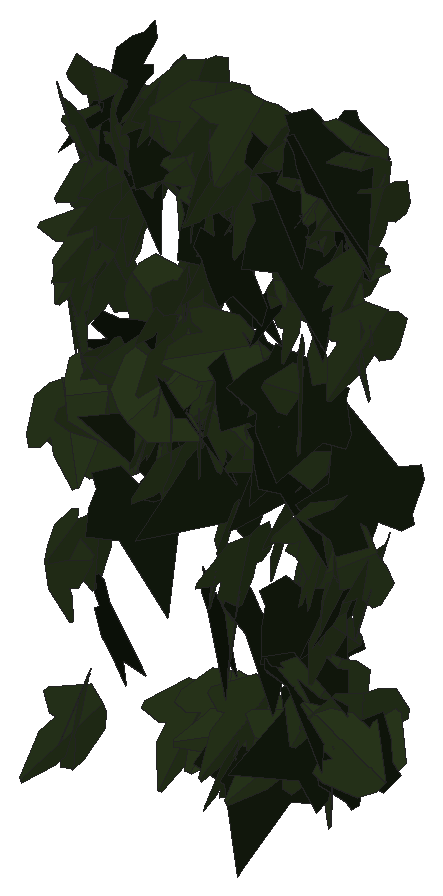
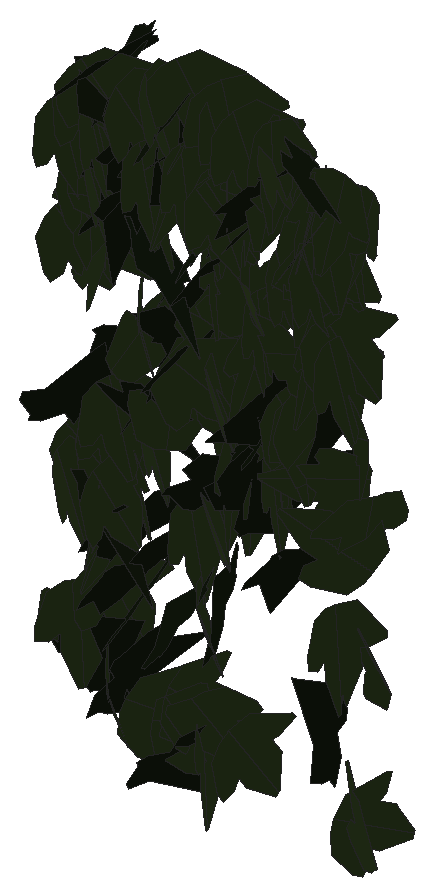
# SketchUp Ruby script. Lengths in inches.
U = 1.inch
M = Sketchup.active_model
def pt(a) = Geom::Point3d.new(a.map { |v| v * U })
def face(e, loops, mat)
  f = e.add_face(loops[0].map { |a| pt(a) })
  loops[1..].each { |l| e.add_face(l.map { |a| pt(a) }).erase! }
  f.material = f.back_material = mat if mat
  f
end
# faces: each face lists its corners as indices into pts; further lists are holes
def faces(e, pts, list, mat = nil) = list.each { |f| face(e, (f[0].is_a?(Array) ? f : [f]).map { |l| l.map { |i| pts[i] } }, mat) }
# xy, xz, yz: faces in a plane at the given z, y or x. An outline is a flat list of corners, or four numbers for a rectangle; further outlines are holes
def ring(l) = l.size == 4 ? [[l[0], l[1]], [l[2], l[1]], [l[2], l[3]], [l[0], l[3]]] : l.each_slice(2).to_a
def flat(e, list, mat, &to3) = list.each { |f| face(e, (f[0].is_a?(Array) ? f : [f]).map { |l| ring(l).map { |u, v| to3.(u, v) } }, mat) }
def xy(e, z, list, mat = nil) = flat(e, list, mat) { |x, y| [x, y, z] }
def xz(e, y, list, mat = nil) = flat(e, list, mat) { |x, z| [x, y, z] }
def yz(e, x, list, mat = nil) = flat(e, list, mat) { |y, z| [x, y, z] }
def lines(e, pts, list) = list.each { |a, b| e.add_line(pt(pts[a]), pt(pts[b])) }
# prism: a flat outline (further loops are holes) pulled along v
def prism(e, loops, v, mat = nil)
  f = face(e, loops, mat); d = Geom::Vector3d.new(v.map { |x| x * U })
  f.pushpull(f.normal.samedirection?(d) ? d.length : -d.length)
end
def box(e, o, s, mat = nil) = prism(e, [[o, [o[0] + s[0], o[1], o[2]], [o[0] + s[0], o[1] + s[1], o[2]], [o[0], o[1] + s[1], o[2]]]], [0, 0, s[2]], mat)
def at(x, y, z, deg = 0) = Geom::Transformation.translation(pt([x, y, z])) * Geom::Transformation.rotation(ORIGIN, Z_AXIS, deg.degrees)
def axes(o, x, y, z) = Geom::Transformation.new([*x, 0, *y, 0, *z, 0, *pt(o).to_a, 1])
def part(name) = M.definitions.add(name)
# library, detail: a bought-in or finely detailed component or shape, given as its bounding box
def library(name, o, s) = part(name).tap { |d| box(d.entities, o, s) }
def detail(e, o, s) = box(e.add_group.entities, o, s)
def put(e, d, t, mat = nil) = e.add_instance(d, t).tap { |i| i.material = mat if mat }
def group(e, t, mat = nil) = e.add_group.tap { |g| g.transformation = t; g.material = mat if mat }.entities
root = M.entities
M.materials.add("efeu1").color = [18, 25, 13]
M.materials.add("efeu2").color = [43, 57, 29]
c1 = part("ivyleaf_10")
p = [[0,0.5,-0.03],[-0.0625,2.02,-0.43],[-0.19,2.01,-0.46],[-0.54,1.05,-0.29],[-0.52,0.625,-0.18],[-0.83,0.76,-0.28],
  [-1.16,0.64,-0.33],[-1.15,0.33,-0.24],[-0.77,-0.39,0.02],[-0.3,-0.51,0.16],[0.04,-0.48,0.23],[-0.02,2.01,-0.4375],
  [-0.06,2.01,-0.43],[0.04,-0.49,0.23],[0.67,-0.49,0.14],[1.38,0.36,-0.2],[1.375,0.51,-0.24],[0.81,0.65,-0.19],
  [0.62,0.59,-0.15],[0.6,1.09,-0.28],[0.5,1.23,-0.31]]
faces(c1.entities,p,[[0,1,2,3,4,5,6,7,8,9,10],[11,12,0,13,14,15,16,17,18,19,20]],"efeu2")
c2 = part("ivyleaf_9")
p = [[1.54,2.16,1.25],[1.36,2.04,1.19],[-0.21,0.99,0.68],[-0.71,1.11,0.82],[-0.85,0.86,0.67],[-0.8,0.17,0.21],
  [-0.9,-0.01,0.1],[-0.67,-0.16,-0.02],[-0.08,-0.08,-0.05],[-0.03,-0.6,-0.4],[0.65,-0.88,-0.66],[0.83,-0.6,-0.49],
  [1.29,-0.42,-0.43],[1.8125,-0.07,-0.26],[1.21,0.44,0.15]]
faces(c2.entities,p,[[0,1,2,3,4,5,6,7,8,9,10,11,12,13,14]],"efeu1")
put(root,c1,axes([13.07,223.93,219.02],[0.34908,0.08349,-0.3481],[0.3274,0.12214,0.35762],[0.14475,-0.47761,0.0306]))
put(root,c2,axes([15.1,224.2,221.98],[-0.02137,-0.46964,-0.17023],[0.02814,0.16899,-0.46974],[0.49875,-0.02966,0.0192]))
put(root,c1,axes([11.76,224.47,214.32],[-0.03853,-0.20251,0.45553],[0.01998,-0.45714,-0.20154],[0.49811,0.00267,0.04332]))
put(root,c1,axes([14.96,224.19,218.31],[0.18515,-0.46397,0.0213],[0.00524,-0.02084,-0.49954],[0.46443,0.1852,-0.00286]))
put(root,c2,axes([14.79,224.2,218.98],[0.26219,-0.42405,-0.03791],[-0.02071,0.03177,-0.49856],[0.42524,0.26301,-0.00091]))
put(root,c2,axes([15.28,224.2,222.875],[0.32575,-0.3792,0.0098],[0.0052,-0.00845,-0.4999],[0.37929,0.32579,-0.00156]))
put(root,c1,axes([14.39,224.26,223.06],[-0.34984,-0.27143,0.23225],[-0.13064,-0.20535,-0.43677],[0.33248,-0.36628,0.07276]))
put(root,c1,axes([14.16,224.2,220.03],[0.19394,0.0032,-0.46085],[-0.4597,-0.03413,-0.19369],[-0.0327,0.49882,-0.0103]))
put(root,c1,axes([12.87,224.29,219.09],[0.37584,-0.28416,0.16732],[0.12516,-0.1118,-0.47099],[0.30509,0.39592,-0.01291]))
put(root,c2,axes([13.68,224.41,216.49],[0.13988,-0.0343,-0.47881],[0.44812,-0.16948,0.14305],[-0.17211,-0.46915,-0.01667]))
put(root,c1,axes([15.14,223.95,221.07],[0.15402,-0.15681,-0.4491],[-0.29345,0.3402,-0.21943],[0.37439,0.33117,0.01276]))
put(root,c1,axes([11.48,224.37,216.3],[0.1403,-0.18208,-0.44403],[0.33778,-0.29116,0.22612],[-0.34091,-0.36342,0.04131]))
put(root,c1,axes([15.47,224.25,218.32],[-0.16,-0.47044,0.05556],[-0.01054,-0.05509,-0.49684],[0.47359,-0.16016,0.00771]))
put(root,c1,axes([15.27,224.18,217.83],[0.33799,-0.34206,-0.13696],[-0.09006,0.10353,-0.4808],[0.35729,0.34968,0.00837]))
put(root,c2,axes([15,224.45,219.68],[-0.32889,-0.37655,0.00676],[-0.00644,-0.00335,-0.49995],[0.37655,-0.32894,-0.00264]))
put(root,c2,axes([13.98,224.1,221.375],[0.33709,-0.29994,-0.21542],[-0.1401,0.166,-0.45035],[0.34167,0.36398,0.02788]))
put(root,c1,axes([15.41,224.36,216.21],[-0.26685,-0.35438,0.23067],[-0.09339,-0.21663,-0.44085],[0.4124,-0.27836,0.04942]))
put(root,c1,axes([13.91,224.38,217.65],[0.29096,-0.37198,0.16423],[0.10235,-0.12843,-0.47226],[0.39353,0.30844,0.00141]))
put(root,c1,axes([15.98,224.3125,215.26],[0.27486,0.21407,0.35865],[-0.28049,-0.22353,0.34837],[0.30949,-0.3927,-0.00279]))
put(root,c1,axes([13.74,224.32,223.02],[-0.29322,-0.39187,0.10229],[-0.00417,-0.12336,-0.48453],[0.40498,-0.28499,0.06908]))
put(root,c2,axes([14.6,224.5,222.41],[0.12659,-0.43266,0.21628],[0.09311,-0.19759,-0.44977],[0.47466,0.15415,0.03054]))
put(root,c1,axes([13.28,224.23,220.375],[0.04579,-0.49298,-0.0698],[0.00656,0.07069,-0.49493],[0.49786,0.04441,0.01295]))
put(root,c1,axes([13.81,224.09,222.38],[0.15065,-0.38885,-0.27586],[-0.05128,0.27441,-0.41481],[0.474,0.15328,0.0428]))
put(root,c1,axes([13.46,224.21,220.4],[-0.11312,-0.46714,0.13779],[0.08053,0.12157,0.47826],[-0.48033,0.13039,0.04774]))
put(root,c1,axes([12.73,224.4375,219.34],[-0.07491,-0.45012,0.20439],[-0.02215,-0.20346,-0.45619],[0.49386,-0.07741,0.01054]))
put(root,c1,axes([13.81,224.3,222.8],[-0.00181,-0.49999,0.00153],[-0.00042,-0.00153,-0.5],[0.5,-0.00181,-0.00041]))
put(root,c1,axes([12.4375,224.29,221.76],[-0.35085,-0.13023,0.33158],[-0.31144,-0.11379,-0.37424],[0.17294,-0.46914,-0.00127]))
put(root,c2,axes([15.02,224.67,215.2],[0.09076,-0.28104,-0.40346],[0.12552,-0.38344,0.29533],[-0.4754,-0.15489,0.00095]))
put(root,c1,axes([13.36,224.21,218.33],[-0.10689,-0.47282,-0.12254],[0.03705,0.11723,-0.48465],[0.48703,-0.11268,0.00997]))
put(root,c1,axes([14.2,224.31,217.41],[-0.03852,-0.49843,-0.0092],[0.00113,0.00914,-0.49992],[0.49851,-0.03853,0.00042]))
put(root,c2,axes([14.83,224.5,216.21],[0.17024,-0.45509,0.11794],[0.0261,-0.11609,-0.48564],[0.4694,0.1715,-0.01577]))
put(root,c1,axes([13.68,224.44,218.96],[-0.09006,-0.04467,-0.48979],[0.41154,-0.27949,-0.05018],[-0.2693,-0.41218,0.08711]))
put(root,c2,axes([15.1,224.29,217.14],[0.07369,-0.42802,-0.24773],[-0.05304,0.24218,-0.4342],[0.49169,0.09027,-0.0097]))
put(root,c1,axes([14.09,224.62,215.23],[-0.05501,-0.30155,0.39502],[0.02432,-0.39859,-0.30089],[0.49637,-0.01389,0.05852]))
put(root,c1,axes([13.35,224.13,219.83],[-0.10307,-0.41364,-0.26129],[0.09995,0.2436,-0.42505],[0.47894,-0.13985,0.03247]))
put(root,c1,axes([15.71,224.53,221.49],[0.00181,-0.42673,0.26057],[0.01559,-0.2604,-0.42656],[0.49975,0.00967,0.01236]))
put(root,c2,axes([12.61,224.41,217.57],[0.03895,-0.47842,-0.13998],[0.01409,0.14141,-0.47938],[0.49828,0.0334,0.02449]))
put(root,c1,axes([14.71,224.41,222.83],[0.13065,-0.4775,0.07016],[0.01626,-0.06828,-0.49505],[0.48235,0.13164,-0.00231]))
put(root,c1,axes([11.8,224.21,222.2],[-0.42339,0.26533,0.01846],[-0.01493,0.01093,-0.49966],[-0.26556,-0.42365,-0.00133]))
put(root,c1,axes([12.44,224.26,221.375],[-0.11146,-0.47749,-0.09786],[0.00368,0.09956,-0.48997],[0.48741,-0.10994,-0.01868]))
put(root,c1,axes([11.99,224.5,220.65],[-0.22928,-0.35897,0.26187],[-0.08028,-0.25637,-0.4217],[0.43702,-0.23542,0.05992]))
put(root,c1,axes([12.41,224.66,219.05],[-0.08888,-0.19424,-0.45208],[-0.1362,-0.43173,0.21227],[-0.47281,0.16088,0.02383]))
put(root,c1,axes([15.88,224.53,220.77],[-0.13693,-0.40243,0.26326],[-0.0645,-0.25588,-0.4247],[0.47654,-0.15026,0.01816]))
put(root,c1,axes([12.91,224.5,222.75],[0.14554,-0.44777,0.16829],[0.04619,-0.16193,-0.47079],[0.47611,0.15259,-0.00577]))
put(root,c2,axes([15.33,224.46,223.08],[0.07842,-0.48579,-0.08863],[0.06513,0.09913,-0.48573],[0.4895,0.06464,0.07883]))
put(root,c1,axes([13.2,224.59,220.94],[0.21535,-0.17607,0.41548],[0.31437,-0.27172,-0.27809],[0.32372,0.38101,-0.00633]))
put(root,c2,axes([13.89,224.66,218.17],[-0.33893,-0.27039,0.24903],[-0.18704,-0.16476,-0.43344],[0.31645,-0.38697,0.01054]))
put(root,c1,axes([14.76,224.5625,219.84],[0.22591,-0.21738,0.3895],[0.32228,-0.2223,-0.31099],[0.30838,0.39157,0.03967]))
put(root,c1,axes([12.68,224.47,220.15],[-0.23664,-0.02364,-0.43982],[0.38833,-0.24681,-0.19566],[-0.20785,-0.4342,0.13517]))
put(root,c1,axes([14.64,224.67,214.92],[-0.13192,-0.20467,0.4367],[-0.07357,-0.43891,-0.22792],[0.47664,-0.12439,0.08568]))
put(root,c1,axes([13.02,224.3,222.42],[-0.43457,-0.24073,-0.05654],[0.04606,0.03353,-0.49674],[0.24295,-0.43695,-0.00697]))
put(root,c1,axes([15.86,224.38,217.85],[-0.27678,-0.01476,0.41614],[-0.40234,-0.11929,-0.27183],[0.10731,-0.48534,0.05416]))
put(root,c1,axes([13.06,224.22,219],[0.36545,-0.23482,-0.2476],[-0.11524,0.25655,-0.4134],[0.32119,0.35923,0.13339]))
put(root,c2,axes([13.0625,224.36,219.25],[0.39008,-0.30923,-0.04709],[-0.03417,0.0327,-0.49776],[0.31092,0.39155,0.00438]))
put(root,c1,axes([14.92,224.63,219.44],[-0.04595,0.29823,0.39868],[0.09084,-0.38864,0.30118],[0.48953,0.10011,-0.01847]))
put(root,c1,axes([11.55,224.48,214.08],[0.25014,-0.39273,-0.18218],[0.11358,-0.1435,0.4653],[-0.41777,-0.27417,0.01742]))
put(root,c1,axes([11.63,224.32,218.4],[0.19669,0.45876,0.0292],[0.01169,0.02676,-0.49915],[-0.45954,0.19704,-0.0002]))
put(root,c1,axes([13.25,224.66,214.9],[-0.13741,-0.37389,0.3022],[0.05814,-0.32492,-0.37556],[0.47722,-0.06807,0.13277]))
put(root,c1,axes([15.61,224.5625,222.62],[-0.15897,-0.43127,0.19681],[-0.03781,-0.19539,-0.45869],[0.47254,-0.16072,0.02951]))
put(root,c2,axes([15.51,224.23,222.64],[-0.20364,0.45648,0.01244],[-0.00547,0.01118,-0.49985],[-0.45662,-0.20371,0.00044]))
put(root,c1,axes([14.93,224.6,222.7],[-0.00767,-0.44717,0.22356],[-0.00255,-0.22354,-0.44724],[0.49993,-0.008,0.00115]))
put(root,c2,axes([12.39,224.21,219.51],[0.43256,0.05246,0.24524],[0.24385,0.02618,-0.43572],[-0.05856,0.49655,-0.00294]))
put(root,c1,axes([13.8,224.34,221.07],[0.04072,-0.47397,-0.15393],[-0.00353,0.15416,-0.47563],[0.49833,0.03982,0.00921]))
put(root,c1,axes([15.46,224.61,222.86],[-0.31299,-0.2872,0.26373],[-0.09033,-0.27558,-0.4073],[0.37932,-0.3026,0.12062]))
put(root,c1,axes([11.51,224.64,219.53],[-0.19426,0.14305,-0.43795],[0.23473,-0.37825,-0.22766],[-0.39644,-0.29405,0.0798]))
put(root,c2,axes([15.57,224.29,217.22],[-0.2818,0.40728,0.06866],[-0.04675,0.05114,-0.49518],[-0.41037,-0.2855,0.00926]))
put(root,c1,axes([15.45,224.18,216.98],[0.07593,-0.32824,-0.36945],[0.05396,0.37705,-0.32391],[0.49125,0.00932,0.09269]))
put(root,c1,axes([14.35,224.63,218.7],[-0.12286,-0.44473,-0.19267],[-0.06173,-0.18278,0.46128],[-0.48072,0.13713,-0.01]))
put(root,c1,axes([15.06,224.18,221.21],[0.01073,-0.13989,0.47991],[0.28537,0.39583,0.109],[-0.41043,0.27156,0.08834]))
put(root,c2,axes([14.93,224.63,221.59],[0.02893,-0.49827,-0.02976],[-0.00521,0.02951,-0.4991],[0.49914,0.02919,-0.00348]))
put(root,c1,axes([12.89,224.56,218.93],[0.43674,-0.21014,0.12288],[0.10673,-0.06154,-0.48458],[0.21879,0.4495,-0.00889]))
put(root,c2,axes([13.16,224.7,218.09],[-0.07589,-0.00901,0.49412],[-0.45574,-0.1921,-0.0735],[0.19116,-0.46154,0.02094]))
put(root,c1,axes([12.25,224.61,221.46],[0.01889,-0.47846,0.14393],[0.00629,-0.14379,-0.47884],[0.4996,0.0199,0.00058]))
put(root,c2,axes([14.95,224.58,216.64],[0.06157,-0.48432,-0.10788],[-0.0192,0.1063,-0.48819],[0.49582,0.06426,-0.00551]))
put(root,c2,axes([15.82,224.36,215.04],[0.07684,0.00598,0.49402],[-0.38099,0.31903,0.05539],[-0.31455,-0.38495,0.05358]))
put(root,c1,axes([15.19,224.54,218.73],[-0.18926,-0.45616,0.07808],[-0.02096,-0.07582,-0.49377],[0.46232,-0.19018,0.00957]))
put(root,c1,axes([12.49,224.48,219.38],[-0.11728,-0.48522,-0.02838],[-0.00332,0.03,-0.49909],[0.48604,-0.11688,-0.01026]))
put(root,c1,axes([14.03,224.7,219.54],[-0.18389,-0.2811,0.37036],[-0.19324,-0.31604,-0.33582],[0.4229,-0.26664,0.00759]))
put(root,c1,axes([12.23,224.49,221.96],[-0.46242,-0.1069,0.15729],[-0.13801,-0.09592,-0.47091],[0.13086,-0.47893,0.0592]))
put(root,c1,axes([15.48,224.53,222.25],[0.09386,-0.49109,-0.0048],[-0.00158,0.00459,-0.49998],[0.49111,0.09387,-0.00069]))
put(root,c1,axes([15.74,224.49,215.85],[-0.2909,-0.40652,0.01087],[-0.00523,-0.00963,-0.49988],[0.40663,-0.29094,0.00135]))
put(root,c1,axes([13.78,224.49,221.9],[0.02652,-0.49668,-0.05103],[0.01089,0.05167,-0.4972],[0.49918,0.02526,0.01356]))
put(root,c1,axes([12.44,224.31,222.34],[-0.17051,0.44273,0.15784],[-0.0954,0.13182,-0.47278],[-0.46025,-0.19134,0.03952]))
put(root,c1,axes([13.75,224.69,216.4],[0.30683,-0.28012,0.27818],[0.21003,-0.1825,-0.41543],[0.33428,0.37179,0.00567]))
put(root,c2,axes([14.14,224.46,219.67],[0.18861,-0.39686,-0.23859],[-0.0668,0.23161,-0.43806],[0.45822,0.19712,0.03435]))
put(root,c1,axes([15.6,224.48,220.88],[-0.14637,0.03623,0.47672],[-0.47421,-0.07442,-0.13995],[0.06081,-0.4931,0.05615]))
put(root,c1,axes([13.64,224.625,219.46],[0.26493,-0.41205,0.10014],[0.05252,-0.08528,-0.48987],[0.42078,0.27008,-0.0019]))
put(root,c1,axes([13.55,224.71,221.98],[-0.17957,-0.39272,0.25204],[-0.0255,-0.2614,-0.42547],[0.46595,-0.16565,0.07385]))
put(root,c1,axes([11.9,224.58,220.36],[-0.00438,-0.49766,0.04815],[0.008,-0.04822,-0.49761],[0.49992,-0.00359,0.00838]))
put(root,c2,axes([14.05,224.8,216.27],[0.10672,-0.41381,0.25956],[0.08911,-0.24473,-0.42681],[0.48028,0.13736,0.02152]))
put(root,c1,axes([14.12,224.76,214.9],[-0.0868,0.00505,0.49238],[-0.29915,-0.39767,-0.04866],[0.39112,-0.30304,0.07206]))
put(root,c1,axes([13.42,224.35,218.87],[0.33574,-0.2714,-0.25223],[-0.07902,0.2801,-0.40657],[0.36199,0.31287,0.14519]))
put(root,c1,axes([12.88,224.48,218.58],[0.11009,-0.47645,-0.10429],[-0.00774,0.10519,-0.48875],[0.48767,0.10923,0.01578]))
put(root,c1,axes([12.91,224.47,222.82],[-0.01427,-0.48916,-0.10257],[0.02573,0.10176,-0.48886],[0.49913,-0.01923,0.02227]))
put(root,c2,axes([14.87,224.6875,218.9375],[-0.49087,-0.09246,-0.02226],[0.02263,0.00008,-0.49949],[0.09237,-0.49138,0.00411]))
put(root,c1,axes([12.33,224.34,220.375],[0.01458,-0.41778,-0.27431],[0.05631,0.27405,-0.4144],[0.49661,-0.01881,0.05504]))
put(root,c1,axes([12.15,224.44,221.49],[-0.35702,-0.31926,-0.14356],[0.1185,0.08272,-0.47866],[0.32938,-0.37581,0.0166]))
put(root,c1,axes([11.97,224.3,218.67],[0.08868,-0.07012,-0.48705],[0.43533,0.2419,0.04444],[0.2294,-0.43193,0.10395]))
put(root,c1,axes([11.92,224.53,216.86],[-0.06824,-0.4924,-0.05375],[0.01374,0.05236,-0.49706],[0.49513,-0.06932,0.00638]))
put(root,c1,axes([14.15,224.55,222.13],[-0.00765,-0.49846,-0.03844],[0.00621,0.03835,-0.49849],[0.4999,-0.0081,0.0056]))
put(root,c2,axes([14.13,224.8,214.57],[-0.15602,-0.47467,0.01844],[-0.00591,-0.01747,-0.49966],[0.475,-0.15614,-0.00016]))
put(root,c1,axes([12.59,224.67,221.36],[0.06257,-0.48326,0.11202],[0.02217,-0.11007,-0.48723],[0.49557,0.06594,0.00766]))
put(root,c2,axes([11.82,224.72,215.625],[0.22344,-0.09479,-0.43714],[0.44482,-0.00432,0.2283],[-0.04705,-0.49091,0.0824]))
put(root,c1,axes([14.3,224.34,221.97],[0.06515,-0.38527,-0.31196],[0.09838,0.31843,-0.37272],[0.48588,-0.01281,0.1173]))
put(root,c1,axes([15.375,224.65,220.7],[-0.25262,0.28903,-0.32038],[0.21447,-0.23804,-0.38385],[-0.37441,-0.33136,-0.00371]))
put(root,c1,axes([13.91,224.45,214.66],[0.10734,-0.4322,-0.22734],[-0.06053,0.2192,-0.4453],[0.48458,0.12311,-0.00526]))
put(root,c2,axes([12.41,224.66,222.83],[-0.43359,0.20792,-0.13699],[0.09118,-0.12338,-0.47588],[-0.23169,-0.43766,0.06908]))
put(root,c2,axes([12.92,224.52,222.35],[0.15698,-0.39794,-0.25885],[-0.0082,0.27033,-0.42054],[0.47465,0.13628,0.07835]))
put(root,c1,axes([14.69,224.6,221.99],[-0.01405,-0.49973,-0.00848],[-0.00041,0.0085,-0.49993],[0.4998,-0.01404,-0.00065]))
put(root,c1,axes([15.02,224.8,215.01],[0.23799,-0.17274,0.40437],[0.32977,-0.23405,-0.29407],[0.29088,0.40667,0.00253]))
put(root,c1,axes([13.21,224.7,222.97],[-0.12207,-0.46776,0.12766],[-0.00204,-0.13114,-0.48249],[0.48487,-0.11831,0.03011]))
put(root,c2,axes([15.06,224.42,221.84],[0.38256,0.12177,-0.29802],[-0.28391,-0.09062,-0.40148],[-0.15178,0.4764,-0.00019]))
put(root,c1,axes([15.45,224.35,217.43],[0.126,-0.34489,-0.33937],[-0.0018,0.35035,-0.35672],[0.48386,0.09112,0.08704]))
put(root,c1,axes([13.77,224.68,215.2],[0.39121,0.21679,-0.22351],[-0.18913,-0.11967,-0.44711],[-0.24736,0.43437,-0.01163]))
put(root,c2,axes([12.23,224.77,221.87],[0.1839,-0.45993,0.06815],[0.01358,-0.06794,-0.49518],[0.46475,0.18398,-0.0125]))
put(root,c1,axes([15.12,224.8,217.68],[-0.03312,-0.43881,0.23738],[0.03223,-0.23929,-0.43784],[0.49786,-0.0137,0.04414]))
put(root,c1,axes([13.43,224.47,218.51],[0.01249,-0.45722,-0.20198],[0.00745,0.20219,-0.45724],[0.49979,0.00841,0.01186]))
put(root,c2,axes([13.53,224.72,221.22],[0.1305,-0.47965,-0.05389],[-0.00811,0.05364,-0.49705],[0.4826,0.13061,0.00622]))
put(root,c2,axes([15.89,224.53,218.33],[-0.39325,-0.28039,0.12937],[0.10685,0.07298,0.48297],[-0.28972,0.4075,0.00252]))
put(root,c1,axes([11.95,224.53,222.52],[-0.49001,0.09762,-0.019],[0.01453,-0.0242,-0.4992],[-0.09839,-0.48978,0.02088]))
put(root,c1,axes([13.57,224.71,221.99],[-0.14192,-0.46145,0.13008],[-0.01794,-0.13046,-0.48235],[0.4791,-0.14158,0.02047]))
put(root,c2,axes([14.7,224.43,220.88],[-0.28035,0.4072,0.07479],[-0.03148,0.06909,-0.4942],[-0.41281,-0.28181,-0.0131]))
put(root,c1,axes([15.375,224.66,221.63],[0.19248,-0.46129,0.01292],[0.00414,-0.01227,-0.49983],[0.46145,0.19252,-0.0009]))
put(root,c1,axes([15.78,224.6875,217.65],[0.15075,-0.47461,0.04489],[0.01064,-0.04372,-0.49797],[0.47661,0.1511,-0.00308]))
put(root,c1,axes([11.76,224.45,217.78],[-0.18213,-0.25447,0.38996],[0.29069,0.26498,0.30868],[-0.36377,0.33916,0.05142]))
put(root,c1,axes([15.81,224.68,222.27],[-0.11229,-0.48202,0.07107],[-0.00922,-0.07082,-0.49487],[0.48714,-0.11245,0.00701]))
